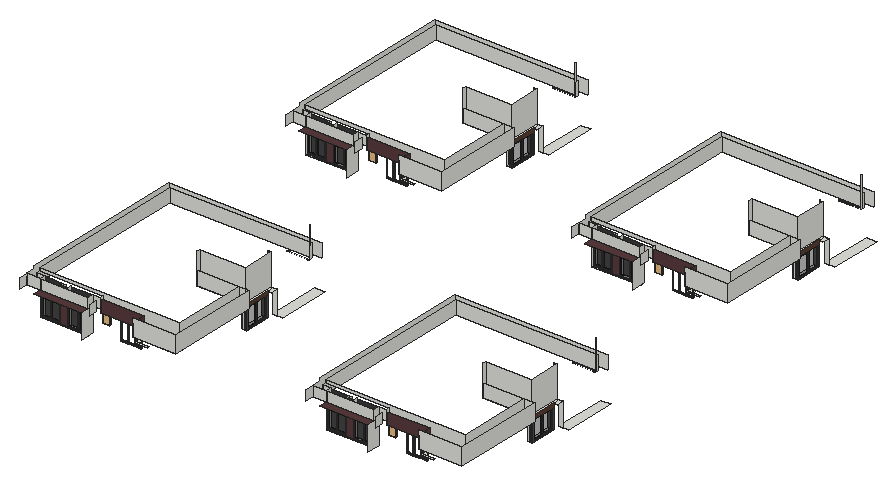
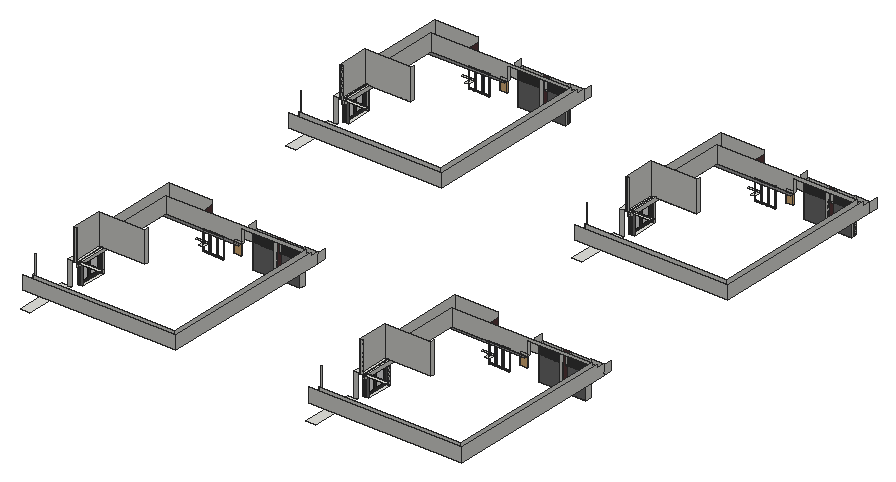
# SketchUp Ruby script. Lengths in inches.
U = 1.inch
M = Sketchup.active_model
def pt(a) = Geom::Point3d.new(a.map { |v| v * U })
def face(e, loops, mat)
  f = e.add_face(loops[0].map { |a| pt(a) })
  loops[1..].each { |l| e.add_face(l.map { |a| pt(a) }).erase! }
  f.material = f.back_material = mat if mat
  f
end
# faces: each face lists its corners as indices into pts; further lists are holes
def faces(e, pts, list, mat = nil) = list.each { |f| face(e, (f[0].is_a?(Array) ? f : [f]).map { |l| l.map { |i| pts[i] } }, mat) }
# xy, xz, yz: faces in a plane at the given z, y or x. An outline is a flat list of corners, or four numbers for a rectangle; further outlines are holes
def ring(l) = l.size == 4 ? [[l[0], l[1]], [l[2], l[1]], [l[2], l[3]], [l[0], l[3]]] : l.each_slice(2).to_a
def flat(e, list, mat, &to3) = list.each { |f| face(e, (f[0].is_a?(Array) ? f : [f]).map { |l| ring(l).map { |u, v| to3.(u, v) } }, mat) }
def xy(e, z, list, mat = nil) = flat(e, list, mat) { |x, y| [x, y, z] }
def xz(e, y, list, mat = nil) = flat(e, list, mat) { |x, z| [x, y, z] }
def yz(e, x, list, mat = nil) = flat(e, list, mat) { |y, z| [x, y, z] }
def lines(e, pts, list) = list.each { |a, b| e.add_line(pt(pts[a]), pt(pts[b])) }
# prism: a flat outline (further loops are holes) pulled along v
def prism(e, loops, v, mat = nil)
  f = face(e, loops, mat); d = Geom::Vector3d.new(v.map { |x| x * U })
  f.pushpull(f.normal.samedirection?(d) ? d.length : -d.length)
end
def box(e, o, s, mat = nil) = prism(e, [[o, [o[0] + s[0], o[1], o[2]], [o[0] + s[0], o[1] + s[1], o[2]], [o[0], o[1] + s[1], o[2]]]], [0, 0, s[2]], mat)
def at(x, y, z, deg = 0) = Geom::Transformation.translation(pt([x, y, z])) * Geom::Transformation.rotation(ORIGIN, Z_AXIS, deg.degrees)
def axes(o, x, y, z) = Geom::Transformation.new([*x, 0, *y, 0, *z, 0, *pt(o).to_a, 1])
def part(name) = M.definitions.add(name)
# library, detail: a bought-in or finely detailed component or shape, given as its bounding box
def library(name, o, s) = part(name).tap { |d| box(d.entities, o, s) }
def detail(e, o, s) = box(e.add_group.entities, o, s)
def put(e, d, t, mat = nil) = e.add_instance(d, t).tap { |i| i.material = mat if mat }
def group(e, t, mat = nil) = e.add_group.tap { |g| g.transformation = t; g.material = mat if mat }.entities
root = M.entities
M.materials.add("Glass_Tinted_Gray").color = [0, 0, 0]
M.materials["Glass_Tinted_Gray"].alpha = 0.125
M.materials.add("Wine2").color = [0, 0, 0]
M.materials["Wine2"].alpha = 0
M.materials.add("[0130_Gainsboro]").color = [39, 45, 50]
M.materials.add("[0135_DarkGray]").color = [81, 81, 81]
M.materials.add("[Color M05]").color = [114, 114, 114]
M.materials.add("[Color M06]").color = [86, 86, 86]
M.materials.add("[Color M07]").color = [58, 58, 58]
M.materials.add("[Granite Brown]").color = [89, 59, 61]
M.materials.add("[Granite Brown]1").color = [89, 63, 50]
M.materials.add("[Mirror 02]").color = [229, 229, 229]
M.materials.add("[Terrazzo Light Blue]").color = [196, 214, 227]
c1 = part("PENTEK_RP Fineline 50S_Sliding_DoorCase_E1")
box(c1.entities,[0,0,0],[1.51,3.66,99.27],"[0135_DarkGray]")
c2 = part("PENTEK_RP Fineline 50S_SlidingDooe_Case_E2")
box(c2.entities,[0,0,0],[96.25,3.66,1.51],"[0135_DarkGray]")
c3 = part("pentek_RP Fineline 50S_SlidingDoor_Case")
put(c3.entities,c1,at(97.76,0,0))
put(c3.entities,c2,at(1.51,0,0))
put(c3.entities,c1,at(0,0,0))
put(c3.entities,c2,at(1.51,0,97.76))
c4 = part("PENTEK_RP Fineline 50S_SlidingDoor_GlazingBead_2")
box(c4.entities,[0,0,0],[0.56,0.59,94.39],"[0135_DarkGray]")
c5 = part("PENTEK_RP Fineline 50S_SlidingDoor_Glass")
box(c5.entities,[0,0,0],[46.58,0.16,94.39],"Glass_Tinted_Gray")
c6 = part("PENTEK_RP Fineline 50S_SlidingDoor_GlazingBead")
box(c6.entities,[0,0,0],[45.47,0.59,0.56],"[0135_DarkGray]")
c7 = part("PENTEK_RP Fineline 50S_SlidingDoor_Leaf_E1")
xy(c7.entities,0,[[0,0,0.93,1.97],[0.93,1.57,1.49,1.97]],"[0135_DarkGray]")
xy(c7.entities,96.25,[[0,0,0.93,0,0.93,1.57,1.49,1.57,1.49,1.97,0,1.97]],"[0135_DarkGray]")
xz(c7.entities,0,[[0,0,0.93,96.25]],"[0135_DarkGray]")
xz(c7.entities,1.57,[[0.93,0,1.49,95.32],[0.93,95.32,1.49,96.25]],"[0135_DarkGray]")
xz(c7.entities,1.97,[[0,0,1.49,96.25]],"[0135_DarkGray]")
yz(c7.entities,0,[[0,0,1.97,96.25]],"[0135_DarkGray]")
yz(c7.entities,0.93,[[0,0,1.57,0.93],[0,0.93,1.57,95.32],[0,95.32,1.57,96.25]],"[0135_DarkGray]")
yz(c7.entities,1.49,[[1.57,0,1.97,95.32],[1.57,95.32,1.97,96.25]],"[0135_DarkGray]")
c8 = part("PENTEK_RP Fineline 50S_SlidingDoor_Leaf_E2")
xy(c8.entities,0,[[0,0,0,1.57,0.56,1.57,0.56,1.97,46.02,1.97,46.02,1.57,46.58,1.57,46.58,0]],"[0135_DarkGray]")
xy(c8.entities,0.93,[[0,0,46.58,1.57]],"[0135_DarkGray]")
xy(c8.entities,1.49,[[0.56,1.57,46.02,1.97]],"[0135_DarkGray]")
xz(c8.entities,0,[[0,0,46.58,0.93]],"[0135_DarkGray]")
xz(c8.entities,1.57,[[0,0,0.56,0.93],[46.02,0,46.58,0.93],[0.56,0.93,46.02,1.49]],"[0135_DarkGray]")
xz(c8.entities,1.97,[[0.56,0,46.02,1.49]],"[0135_DarkGray]")
yz(c8.entities,0,[[0,0,1.57,0.93]],"[0135_DarkGray]")
yz(c8.entities,0.56,[[1.57,0,1.97,0.93],[1.57,0.93,1.97,1.49]],"[0135_DarkGray]")
yz(c8.entities,46.02,[[1.57,0,1.97,0.93],[1.57,0.93,1.97,1.49]],"[0135_DarkGray]")
yz(c8.entities,46.58,[[0,0,1.57,0.93]],"[0135_DarkGray]")
c9 = part("PENTEK_RP Fineline S_SlidingDoor_Leaf1")
put(c9.entities,c4,at(0.93,0,0.93))
put(c9.entities,c4,at(46.96,0,0.93))
put(c9.entities,c5,at(1.49,1.42,0.93))
put(c9.entities,c6,at(1.49,0,0.93))
put(c9.entities,c5,at(1.49,0.59,0.93),"[Terrazzo Light Blue]")
put(c9.entities,c7,at(0,0,0))
put(c9.entities,c7,axes([48.44,0,0],[-1,0,0],[0,1,0],[0,0,1]))
put(c9.entities,c8,axes([0.93,0,96.25],[1,0,0],[0,1,0],[0,0,-1]))
put(c9.entities,c8,at(0.93,0,0))
put(c9.entities,c6,at(1.49,0,94.77))
c10 = part("PENTEK_RP Fineline 50S_SlidingDoor_Leaf2")
put(c10.entities,c5,at(1.49,1.42,0.93))
put(c10.entities,c6,at(1.49,0,94.77))
put(c10.entities,c4,at(46.96,0,0.93))
put(c10.entities,c5,at(1.49,0.59,0.93),"[Mirror 02]")
put(c10.entities,c4,at(0.93,0,0.93))
put(c10.entities,c7,at(0,0,0))
put(c10.entities,c7,axes([48.44,0,0],[-1,0,0],[0,1,0],[0,0,1]))
put(c10.entities,c6,at(1.49,0,0.93))
put(c10.entities,c8,axes([0.93,0,96.25],[1,0,0],[0,1,0],[0,0,-1]))
put(c10.entities,c8,at(0.93,0,0))
c11 = part("PENTEK - Slimmest Steel Sliding Door / Window\#1")
put(c11.entities,c3,at(0,-1.88,-0.09))
put(c11.entities,c9,at(1.51,-2.27,1.42))
put(c11.entities,c10,at(49.32,-0.3,1.42))
c12 = part("Framed glazing panel")
xy(c12.entities,0,[[0,-0.98,43.07,0],[0,0,43.07,1.4]],"[0130_Gainsboro]")
xy(c12.entities,0.3,[[0.3,-1.43,42.77,-0.98]],"[0130_Gainsboro]")
xy(c12.entities,2.95,[[2.95,-1.43,40.12,-0.63],[2.95,-0.63,40.12,0],[2.95,0,40.12,0.64],[2.95,0.64,40.12,1.4]],"[0130_Gainsboro]")
xy(c12.entities,3.54,[[3.54,-0.63,39.53,0],[3.54,0,39.53,0.64]],"[0130_Gainsboro]")
xy(c12.entities,111.8125,[[3.54,-0.63,39.53,0],[3.54,0,39.53,0.64]],"[0130_Gainsboro]")
xy(c12.entities,112.4,[[2.95,-1.43,40.12,-0.63],[2.95,-0.63,40.12,0],[2.95,0,40.12,0.64],[2.95,0.64,40.12,1.4]],"[0130_Gainsboro]")
xy(c12.entities,115.05,[[0.3,-1.43,42.77,-0.98]],"[0130_Gainsboro]")
xy(c12.entities,115.35,[[0,-0.98,43.07,0],[0,0,43.07,1.4]],"[0130_Gainsboro]")
xz(c12.entities,-1.43,[[[0.3,0.3,42.77,115.05],[2.95,2.95,40.12,112.4]]],"[0130_Gainsboro]")
xz(c12.entities,-0.98,[[[0,0,43.07,115.35],[0.3,0.3,42.77,115.05]]],"[0130_Gainsboro]")
xz(c12.entities,-0.63,[[[2.95,2.95,40.12,112.4],[3.54,3.54,39.53,111.8125]]],"[0130_Gainsboro]")
xz(c12.entities,0,[[3.54,3.54,39.53,111.8125]],"Wine2")
xz(c12.entities,0,[[[0,0,43.07,115.35],[2.95,2.95,40.12,112.4]],[[2.95,2.95,40.12,112.4],[3.54,3.54,39.53,111.8125]]],"[0130_Gainsboro]")
xz(c12.entities,0.64,[[[2.95,2.95,40.12,112.4],[3.54,3.54,39.53,111.8125]]],"[0130_Gainsboro]")
xz(c12.entities,1.4,[[[0,0,43.07,115.35],[2.95,2.95,40.12,112.4]]],"[0130_Gainsboro]")
yz(c12.entities,0,[[-0.98,0,0,115.35],[0,0,1.4,115.35]],"[0130_Gainsboro]")
yz(c12.entities,0.3,[[-1.43,0.3,-0.98,115.05]],"[0130_Gainsboro]")
yz(c12.entities,2.95,[[-1.43,2.95,-0.63,112.4],[-0.63,2.95,0,112.4],[0,2.95,0.64,112.4],[0.64,2.95,1.4,112.4]],"[0130_Gainsboro]")
yz(c12.entities,3.54,[[-0.63,3.54,0,111.8125],[0,3.54,0.64,111.8125]],"[0130_Gainsboro]")
yz(c12.entities,39.53,[[-0.63,3.54,0,111.8125],[0,3.54,0.64,111.8125]],"[0130_Gainsboro]")
yz(c12.entities,40.12,[[-1.43,2.95,-0.63,112.4],[-0.63,2.95,0,112.4],[0,2.95,0.64,112.4],[0.64,2.95,1.4,112.4]],"[0130_Gainsboro]")
yz(c12.entities,42.77,[[-1.43,0.3,-0.98,115.05]],"[0130_Gainsboro]")
yz(c12.entities,43.07,[[-0.98,0,0,115.35],[0,0,1.4,115.35]],"[0130_Gainsboro]")
c13 = part("Glazed panel assembly")
put(c13.entities,c12,axes([90.57,1.43,0],[1.05148,0,0],[0,1,0],[0,0,1]))
put(c13.entities,c12,axes([0,1.43,0],[1.05148,0,0],[0,1,0],[0,0,1]))
put(c13.entities,c12,axes([45.29,1.43,0],[1.05148,0,0],[0,1,0],[0,0,1]))
c14 = library("Klein+raam",[128.36,12.7,0],[19.68,5.51,55.12])
xy(root,1659.3125,[[319.53,1799.9375,523.04,1799.9375,523.04,1822.9375,431.33,1822.9375,431.33,1806.5625,406.84,1806.5625,406.84,1822.9375,319.53,1822.9375],[1537.72,1799.9375,1741.23,1799.9375,1741.23,1822.9375,1649.52,1822.9375,1649.52,1806.5625,1625.03,1806.5625,1625.03,1822.9375,1537.72,1822.9375],[319.53,3214.625,523.04,3214.625,523.04,3237.625,431.33,3237.625,431.33,3221.25,406.84,3221.25,406.84,3237.625,319.53,3237.625],[1537.72,3214.625,1741.23,3214.625,1741.23,3237.625,1649.52,3237.625,1649.52,3221.25,1625.03,3221.25,1625.03,3237.625,1537.72,3237.625]])
xy(root,1661.36,[[890.875,2156.01,913.875,2266.33],[2109.0625,2156.01,2132.0625,2266.33],[890.875,3570.7,913.875,3681.01],[2109.0625,3570.7,2132.0625,3681.01]])
xy(root,1663.0625,[[913.875,2295.875,954.6875,2518.89],[2132.0625,2295.875,2172.875,2518.89],[913.875,3710.5625,954.6875,3933.57],[2132.0625,3710.5625,2172.875,3933.57]])
xy(root,1693.1875,[[709.36,1814.25,764.59,1822.9375],[1927.54,1814.25,1982.78,1822.9375],[709.01,1822.9375,727.9,1851.6875],[1927.2,1822.9375,1946.09,1851.6875],[709.36,3228.9375,764.59,3237.625],
  [1927.54,3228.9375,1982.78,3237.625],[709.01,3237.625,727.9,3266.375],[1927.2,3237.625,1946.09,3266.375]])
xy(root,1747,[[894.3125,2107.9375,913.875,2148.625],[2112.5,2107.9375,2132.0625,2148.625],[894.3125,3522.625,913.875,3563.3125],[2112.5,3522.625,2132.0625,3563.3125]])
xy(root,1747.04,[[894.3125,2148.83,913.875,2156.01],[2112.5,2148.83,2132.0625,2156.01],[890.875,2156.01,913.875,2266.33],[2109.0625,2156.01,2132.0625,2266.33],[894.3125,3563.51,913.875,3570.7],
  [2112.5,3563.51,2132.0625,3570.7],[890.875,3570.7,913.875,3681.01],[2109.0625,3570.7,2132.0625,3681.01]])
xy(root,1749.375,[[883.05,1851.6875,894.3125,2295.875],[2101.24,1851.6875,2112.5,2295.875],[883.05,3266.375,894.3125,3710.5625],[2101.24,3266.375,2112.5,3710.5625]])
xy(root,1749.375,[[557.88,1835.8125,883.05,1851.6875],[1776.07,1835.8125,2101.24,1851.6875],[557.88,3250.5,883.05,3266.375],[1776.07,3250.5,2101.24,3266.375]],"[Color M05]")
xy(root,1749.375,[[741.54,1763.25,925.6875,1799.9375],[1959.73,1763.25,2143.875,1799.9375],[741.54,1799.9375,925.6875,1822.9375],[1959.73,1799.9375,2143.875,1822.9375],[557.88,1822.9375,557.88,1835.8125,883.05,1835.8125,883.05,1851.6875,894.3125,1851.6875,894.3125,2148.83,925.6875,2148.83,925.6875,1822.9375],
  [1776.07,1822.9375,1776.07,1835.8125,2101.24,1835.8125,2101.24,1851.6875,2112.5,1851.6875,2112.5,2148.83,2143.875,2148.83,2143.875,1822.9375],[557.4,1835.1875,557.88,1835.8125],[1775.59,1835.1875,1776.07,1835.8125],[741.54,3177.9375,925.6875,3214.625],[1959.73,3177.9375,2143.875,3214.625],
  [741.54,3214.625,925.6875,3237.625],[1959.73,3214.625,2143.875,3237.625],[557.88,3237.625,557.88,3250.5,883.05,3250.5,883.05,3266.375,894.3125,3266.375,894.3125,3563.51,925.6875,3563.51,925.6875,3237.625],[1776.07,3237.625,1776.07,3250.5,2101.24,3250.5,2101.24,3266.375,2112.5,3266.375,2112.5,3563.51,2143.875,3563.51,2143.875,3237.625],[557.4,3249.875,557.88,3250.5],
  [1775.59,3249.875,1776.07,3250.5]],"[Color M06]")
xy(root,1749.375,[[557.4,1822.9375,557.88,1835.1875],[1775.59,1822.9375,1776.07,1835.1875],[557.4,3237.625,557.88,3249.875],[1775.59,3237.625,1776.07,3249.875]],"[Granite Brown]")
xy(root,1764,[[890.875,1835.8125,894.3125,2148.83],[2109.0625,1835.8125,2112.5,2148.83],[708.18,2148.83,883.05,2162.73],[883.05,2148.83,890.875,2162.73],[890.875,2148.83,894.3125,2162.73],
  [894.3125,2148.83,913.875,2148.83,913.875,2295.875,903.5,2295.875,903.5,2162.73,894.3125,2162.73],[1926.36,2148.83,2101.24,2162.73],[2101.24,2148.83,2109.0625,2162.73],[2109.0625,2148.83,2112.5,2162.73],[2112.5,2148.83,2132.0625,2148.83,2132.0625,2295.875,2121.6875,2295.875,2121.6875,2162.73,2112.5,2162.73],
  [883.05,2162.73,890.875,2278.25],[890.875,2162.73,894.3125,2295.875],[894.3125,2162.73,903.5,2295.875],[2101.24,2162.73,2109.0625,2278.25],[2109.0625,2162.73,2112.5,2295.875],
  [2112.5,2162.73,2121.6875,2295.875],[913.875,2266.33,930.75,2295.875],[2132.0625,2266.33,2148.9375,2295.875],[795.3125,2278.25,883.05,2284.4375],[883.05,2278.25,890.875,2284.4375],
  [2013.5,2278.25,2101.24,2284.4375],[2101.24,2278.25,2109.0625,2284.4375],[795.3125,2284.4375,883.05,2295.875],[883.05,2284.4375,890.875,2295.875],[2013.5,2284.4375,2101.24,2295.875],
  [2101.24,2284.4375,2109.0625,2295.875],[795.3125,2517.14,890.875,2518.89],[2013.5,2517.14,2109.0625,2518.89],[890.875,3250.5,894.3125,3563.51],[2109.0625,3250.5,2112.5,3563.51],
  [708.18,3563.51,883.05,3577.41],[883.05,3563.51,890.875,3577.41],[890.875,3563.51,894.3125,3577.41],[894.3125,3563.51,913.875,3563.51,913.875,3710.5625,903.5,3710.5625,903.5,3577.41,894.3125,3577.41],[1926.36,3563.51,2101.24,3577.41],
  [2101.24,3563.51,2109.0625,3577.41],[2109.0625,3563.51,2112.5,3577.41],[2112.5,3563.51,2132.0625,3563.51,2132.0625,3710.5625,2121.6875,3710.5625,2121.6875,3577.41,2112.5,3577.41],[883.05,3577.41,890.875,3692.9375],[890.875,3577.41,894.3125,3710.5625],
  [894.3125,3577.41,903.5,3710.5625],[2101.24,3577.41,2109.0625,3692.9375],[2109.0625,3577.41,2112.5,3710.5625],[2112.5,3577.41,2121.6875,3710.5625],[913.875,3681.01,930.75,3710.5625],
  [2132.0625,3681.01,2148.9375,3710.5625],[795.3125,3692.9375,883.05,3699.125],[883.05,3692.9375,890.875,3699.125],[2013.5,3692.9375,2101.24,3699.125],[2101.24,3692.9375,2109.0625,3699.125],
  [795.3125,3699.125,883.05,3710.5625],[883.05,3699.125,890.875,3710.5625],[2013.5,3699.125,2101.24,3710.5625],[2101.24,3699.125,2109.0625,3710.5625],[795.3125,3931.82,890.875,3933.57],
  [2013.5,3931.82,2109.0625,3933.57]])
xy(root,1764,[[319.53,1763.25,523.04,1799.9375],[1537.72,1763.25,1741.23,1799.9375],[319.53,3177.9375,523.04,3214.625],[1537.72,3177.9375,1741.23,3214.625]],"[Granite Brown]")
xz(root,1763.25,[[741.54,1749.375,925.6875,1821.625],[1959.73,1749.375,2143.875,1821.625]])
xz(root,1763.25,[[557.4,1764,557.88,1801.625],[1775.59,1764,1776.07,1801.625]],"[Granite Brown]")
xz(root,1799.9375,[[262.875,1764,319.53,1807.33],[319.53,1764,523.04,1805.3125],[1481.0625,1764,1537.72,1807.33],[1537.72,1764,1741.23,1805.3125]])
xz(root,1806.5625,[[406.84,1659.3125,431.33,1659.3125,431.33,1808.75,407.44,1808.75,407.44,1805.3125,396.84,1805.37,396.63,1764.05,396.11,1659.37],[1625.03,1659.3125,1649.52,1659.3125,1649.52,1808.75,1625.63,1808.75,1625.63,1805.3125,1615.02,1805.37,1614.82,1764.05,1614.29,1659.37]],"[Granite Brown]")
xz(root,1822.9375,[[285.875,1764,319.53,1807.33],[396.63,1764,396.84,1764.05],[396.84,1764,396.84,1764.05,407.44,1764],[407.44,1764,396.84,1764.05,396.84,1805.37,407.44,1805.3125],[407.44,1764,407.44,1805.3125,407.65,1805.3125],
  [523.04,1764,557.4,1805.3125],[1504.0625,1764,1537.72,1807.33],[1614.82,1764,1615.02,1764.05],[1615.02,1764,1615.02,1764.05,1625.63,1764],[1625.63,1764,1615.02,1764.05,1615.02,1805.37,1625.63,1805.3125],
  [1625.63,1764,1625.63,1805.3125,1625.84,1805.3125],[1741.23,1764,1775.59,1805.3125],[396.63,1764.05,396.84,1805.37,396.84,1764.05],[1614.82,1764.05,1615.02,1805.37,1615.02,1764.05]])
xz(root,1822.9375,[[319.53,1659.3125,396.11,1659.3125,396.63,1764,319.53,1764],[431.33,1659.3125,523.04,1764],[1537.72,1659.3125,1614.29,1659.3125,1614.82,1764,1537.72,1764],[1649.52,1659.3125,1741.23,1764]],"[Color M05]")
xz(root,1822.9375,[[319.53,1764,319.53,1805.37,396.84,1805.37,396.63,1764.05,396.63,1764],[431.33,1764,523.04,1805.3125],[1537.72,1764,1537.72,1805.37,1615.02,1805.37,1614.82,1764.05,1614.82,1764],[1649.52,1764,1741.23,1805.3125]],"[Color M07]")
xz(root,1822.9375,[[557.4,1749.375,557.88,1764],[557.88,1749.375,741.54,1801.625],[1775.59,1749.375,1776.07,1764],[1776.07,1749.375,1959.73,1801.625],[557.4,1764,557.88,1801.625],
  [1775.59,1764,1776.07,1801.625]],"[Granite Brown]")
xz(root,1835.1875,[[556.34,1706.43,557.4,1758.71],[1774.53,1706.43,1775.59,1758.71]])
xz(root,1835.8125,[[557.4,1749.375,557.4,1807.33,285.875,1807.33,285.875,1821.625,883.05,1821.625,883.05,1749.375],[1775.59,1749.375,1775.59,1807.33,1504.0625,1807.33,1504.0625,1821.625,2101.24,1821.625,2101.24,1749.375]])
xz(root,2148.83,[[894.3125,1747.04,913.875,1749.375],[2112.5,1747.04,2132.0625,1749.375],[913.875,1749.375,925.6875,1764],[2132.0625,1749.375,2143.875,1764],[708.18,1764,883.05,1821.625],
  [883.05,1764,913.875,1821.625],[913.875,1764,925.6875,1821.625],[1926.36,1764,2101.24,1821.625],[2101.24,1764,2132.0625,1821.625],[2132.0625,1764,2143.875,1821.625]])
xz(root,2156.01,[[890.875,1661.36,894.3125,1747.04],[894.3125,1661.36,913.875,1747.04],[2109.0625,1661.36,2112.5,1747.04],[2112.5,1661.36,2132.0625,1747.04]])
xz(root,2162.73,[[708.18,1764,903.5,1895.25],[1926.36,1764,2121.6875,1895.25]])
xz(root,2266.33,[[890.875,1661.36,913.875,1747.04],[2109.0625,1661.36,2132.0625,1747.04]],"[Color M05]")
xz(root,2295.875,[[913.875,1663.0625,930.75,1764],[2132.0625,1663.0625,2148.9375,1764],[883.05,1749.375,890.875,1764],[890.875,1749.375,894.3125,1764],[2101.24,1749.375,2109.0625,1764],
  [2109.0625,1749.375,2112.5,1764],[890.875,1764,894.3125,1895.25],[894.3125,1764,903.5,1895.25],[2109.0625,1764,2112.5,1895.25],[2112.5,1764,2121.6875,1895.25]])
xz(root,2531.375,[[285.875,1764,890.875,1821.625],[1504.0625,1764,2109.0625,1821.625]])
xz(root,2554.375,[[262.875,1764,913.875,1821.625],[1481.0625,1764,2132.0625,1821.625]])
xz(root,3177.9375,[[741.54,1749.375,925.6875,1821.625],[1959.73,1749.375,2143.875,1821.625]])
xz(root,3177.9375,[[557.4,1764,557.88,1801.625],[1775.59,1764,1776.07,1801.625]],"[Granite Brown]")
xz(root,3214.625,[[262.875,1764,319.53,1807.33],[319.53,1764,523.04,1805.3125],[1481.0625,1764,1537.72,1807.33],[1537.72,1764,1741.23,1805.3125]])
xz(root,3221.25,[[406.84,1659.3125,431.33,1659.3125,431.33,1808.75,407.44,1808.75,407.44,1805.3125,396.84,1805.37,396.63,1764.05,396.11,1659.37],[1625.03,1659.3125,1649.52,1659.3125,1649.52,1808.75,1625.63,1808.75,1625.63,1805.3125,1615.02,1805.37,1614.82,1764.05,1614.29,1659.37]],"[Granite Brown]")
xz(root,3237.625,[[285.875,1764,319.53,1807.33],[396.63,1764,396.84,1764.05],[396.84,1764,396.84,1764.05,407.44,1764],[407.44,1764,396.84,1764.05,396.84,1805.37,407.44,1805.3125],[407.44,1764,407.44,1805.3125,407.65,1805.3125],
  [523.04,1764,557.4,1805.3125],[1504.0625,1764,1537.72,1807.33],[1614.82,1764,1615.02,1764.05],[1615.02,1764,1615.02,1764.05,1625.63,1764],[1625.63,1764,1615.02,1764.05,1615.02,1805.37,1625.63,1805.3125],
  [1625.63,1764,1625.63,1805.3125,1625.84,1805.3125],[1741.23,1764,1775.59,1805.3125],[396.63,1764.05,396.84,1805.37,396.84,1764.05],[1614.82,1764.05,1615.02,1805.37,1615.02,1764.05]])
xz(root,3237.625,[[319.53,1659.3125,396.11,1659.3125,396.63,1764,319.53,1764],[431.33,1659.3125,523.04,1764],[1537.72,1659.3125,1614.29,1659.3125,1614.82,1764,1537.72,1764],[1649.52,1659.3125,1741.23,1764]],"[Color M05]")
xz(root,3237.625,[[319.53,1764,319.53,1805.37,396.84,1805.37,396.63,1764.05,396.63,1764],[431.33,1764,523.04,1805.3125],[1537.72,1764,1537.72,1805.37,1615.02,1805.37,1614.82,1764.05,1614.82,1764],[1649.52,1764,1741.23,1805.3125]],"[Color M07]")
xz(root,3237.625,[[557.4,1749.375,557.88,1764],[557.88,1749.375,741.54,1801.625],[1775.59,1749.375,1776.07,1764],[1776.07,1749.375,1959.73,1801.625],[557.4,1764,557.88,1801.625],
  [1775.59,1764,1776.07,1801.625]],"[Granite Brown]")
xz(root,3249.875,[[556.34,1706.43,557.4,1758.71],[1774.53,1706.43,1775.59,1758.71]])
xz(root,3250.5,[[557.4,1749.375,557.4,1807.33,285.875,1807.33,285.875,1821.625,883.05,1821.625,883.05,1749.375],[1775.59,1749.375,1775.59,1807.33,1504.0625,1807.33,1504.0625,1821.625,2101.24,1821.625,2101.24,1749.375]])
xz(root,3563.51,[[894.3125,1747.04,913.875,1749.375],[2112.5,1747.04,2132.0625,1749.375],[913.875,1749.375,925.6875,1764],[2132.0625,1749.375,2143.875,1764],[708.18,1764,883.05,1821.625],
  [883.05,1764,913.875,1821.625],[913.875,1764,925.6875,1821.625],[1926.36,1764,2101.24,1821.625],[2101.24,1764,2132.0625,1821.625],[2132.0625,1764,2143.875,1821.625]])
xz(root,3570.7,[[890.875,1661.36,894.3125,1747.04],[894.3125,1661.36,913.875,1747.04],[2109.0625,1661.36,2112.5,1747.04],[2112.5,1661.36,2132.0625,1747.04]])
xz(root,3577.41,[[708.18,1764,903.5,1895.25],[1926.36,1764,2121.6875,1895.25]])
xz(root,3681.01,[[890.875,1661.36,913.875,1747.04],[2109.0625,1661.36,2132.0625,1747.04]],"[Color M05]")
xz(root,3710.5625,[[913.875,1663.0625,930.75,1764],[2132.0625,1663.0625,2148.9375,1764],[883.05,1749.375,890.875,1764],[890.875,1749.375,894.3125,1764],[2101.24,1749.375,2109.0625,1764],
  [2109.0625,1749.375,2112.5,1764],[890.875,1764,894.3125,1895.25],[894.3125,1764,903.5,1895.25],[2109.0625,1764,2112.5,1895.25],[2112.5,1764,2121.6875,1895.25]])
xz(root,3946.0625,[[285.875,1764,890.875,1821.625],[1504.0625,1764,2109.0625,1821.625]])
xz(root,3969.0625,[[262.875,1764,913.875,1821.625],[1481.0625,1764,2132.0625,1821.625]])
yz(root,262.875,[[1763.25,1764,1799.9375,1805.3125],[1799.9375,1764,1799.9375,1807.33,1835.8125,1807.33,1835.8125,1821.625,2554.375,1821.625,2554.375,1764],[3177.9375,1764,3214.625,1805.3125],[3214.625,1764,3214.625,1807.33,3250.5,1807.33,3250.5,1821.625,3969.0625,1821.625,3969.0625,1764]])
yz(root,285.875,[[1822.9375,1764,2531.375,1764,2531.375,1821.625,1835.8125,1821.625,1835.8125,1807.33,1822.9375,1807.33],[3237.625,1764,3946.0625,1764,3946.0625,1821.625,3250.5,1821.625,3250.5,1807.33,3237.625,1807.33]])
yz(root,319.53,[[1799.9375,1659.3125,1822.9375,1764],[3214.625,1659.3125,3237.625,1764],[1799.9375,1764,1822.9375,1807.33],[3214.625,1764,3237.625,1807.33]])
yz(root,431.33,[[1806.5625,1659.3125,1822.9375,1808.75],[3221.25,1659.3125,3237.625,1808.75]])
yz(root,523.04,[[1763.25,1659.3125,1822.9375,1764],[3177.9375,1659.3125,3237.625,1764],[1799.9375,1764,1822.9375,1805.3125],[3214.625,1764,3237.625,1805.3125]])
yz(root,557.22,[[1763.25,1764,1799.9375,1805.3125],[3177.9375,1764,3214.625,1805.3125]])
yz(root,557.4,[[1822.9375,1749.375,1835.8125,1807.33],[3237.625,1749.375,3250.5,1807.33]])
yz(root,708.18,[[2148.83,1764,2162.73,1895.25],[3563.51,1764,3577.41,1895.25]])
yz(root,741.54,[[1763.25,1749.375,1799.9375,1801.625],[1799.9375,1749.375,1822.9375,1801.625],[3177.9375,1749.375,3214.625,1801.625],[3214.625,1749.375,3237.625,1801.625]],"[Granite Brown]")
yz(root,883.05,[[1835.8125,1749.375,1835.8125,1821.625,2148.83,1821.625,2148.83,1764,2295.875,1764,2295.875,1749.375],[3250.5,1749.375,3250.5,1821.625,3563.51,1821.625,3563.51,1764,3710.5625,1764,3710.5625,1749.375]])
yz(root,890.875,[[2517.14,1764,2518.89,1895.25],[2518.89,1764,2531.375,1821.625],[3931.82,1764,3933.57,1895.25],[3933.57,1764,3946.0625,1821.625]])
yz(root,894.3125,[[2148.83,1749.375,2295.875,1764],[3563.51,1749.375,3710.5625,1764]])
yz(root,903.5,[[2162.73,1764,2295.875,1895.25],[3577.41,1764,3710.5625,1895.25]])
yz(root,913.875,[[2148.83,1747.04,2266.33,1764],[3563.51,1747.04,3681.01,1764]],"[Granite Brown]1")
yz(root,925.6875,[[1763.25,1749.375,2148.83,1821.625],[3177.9375,1749.375,3563.51,1821.625]])
yz(root,1481.0625,[[1763.25,1764,1799.9375,1805.3125],[1799.9375,1764,1799.9375,1807.33,1835.8125,1807.33,1835.8125,1821.625,2554.375,1821.625,2554.375,1764],[3177.9375,1764,3214.625,1805.3125],[3214.625,1764,3214.625,1807.33,3250.5,1807.33,3250.5,1821.625,3969.0625,1821.625,3969.0625,1764]])
yz(root,1504.0625,[[1822.9375,1764,2531.375,1764,2531.375,1821.625,1835.8125,1821.625,1835.8125,1807.33,1822.9375,1807.33],[3237.625,1764,3946.0625,1764,3946.0625,1821.625,3250.5,1821.625,3250.5,1807.33,3237.625,1807.33]])
yz(root,1537.72,[[1799.9375,1659.3125,1822.9375,1764],[3214.625,1659.3125,3237.625,1764],[1799.9375,1764,1822.9375,1807.33],[3214.625,1764,3237.625,1807.33]])
yz(root,1649.52,[[1806.5625,1659.3125,1822.9375,1808.75],[3221.25,1659.3125,3237.625,1808.75]])
yz(root,1741.23,[[1763.25,1659.3125,1822.9375,1764],[3177.9375,1659.3125,3237.625,1764],[1799.9375,1764,1822.9375,1805.3125],[3214.625,1764,3237.625,1805.3125]])
yz(root,1775.4,[[1763.25,1764,1799.9375,1805.3125],[3177.9375,1764,3214.625,1805.3125]])
yz(root,1775.59,[[1822.9375,1749.375,1835.8125,1807.33],[3237.625,1749.375,3250.5,1807.33]])
yz(root,1926.36,[[2148.83,1764,2162.73,1895.25],[3563.51,1764,3577.41,1895.25]])
yz(root,1959.73,[[1763.25,1749.375,1799.9375,1801.625],[1799.9375,1749.375,1822.9375,1801.625],[3177.9375,1749.375,3214.625,1801.625],[3214.625,1749.375,3237.625,1801.625]],"[Granite Brown]")
yz(root,2101.24,[[1835.8125,1749.375,1835.8125,1821.625,2148.83,1821.625,2148.83,1764,2295.875,1764,2295.875,1749.375],[3250.5,1749.375,3250.5,1821.625,3563.51,1821.625,3563.51,1764,3710.5625,1764,3710.5625,1749.375]])
yz(root,2109.0625,[[2517.14,1764,2518.89,1895.25],[2518.89,1764,2531.375,1821.625],[3931.82,1764,3933.57,1895.25],[3933.57,1764,3946.0625,1821.625]])
yz(root,2112.5,[[2148.83,1749.375,2295.875,1764],[3563.51,1749.375,3710.5625,1764]])
yz(root,2121.6875,[[2162.73,1764,2295.875,1895.25],[3577.41,1764,3710.5625,1895.25]])
yz(root,2132.0625,[[2148.83,1747.04,2266.33,1764],[3563.51,1747.04,3681.01,1764]],"[Granite Brown]1")
yz(root,2143.875,[[1763.25,1749.375,2148.83,1821.625],[3177.9375,1749.375,3563.51,1821.625]])
p = [[396.63,1822.9375,1764.05],[396.63,1806.5625,1764.05],[396.84,1806.5625,1805.37],[396.84,1822.9375,1805.37],[1614.82,1822.9375,1764.05],[1614.82,1806.5625,1764.05],
  [1615.02,1806.5625,1805.37],[1615.02,1822.9375,1805.37],[396.63,3237.625,1764.05],[396.63,3221.25,1764.05],[396.84,3221.25,1805.37],[396.84,3237.625,1805.37],
  [1614.82,3237.625,1764.05],[1614.82,3221.25,1764.05],[1615.02,3221.25,1805.37],[1615.02,3237.625,1805.37],[1806.84,1835.1875,1706.43],[1806.84,1835.1875,1758.71],
  [1775.59,1835.1875,1706.43],[1775.59,1835.1875,1758.71],[1625.63,1806.5625,1764],[1625.63,1822.9375,1764],[588.66,1835.1875,1706.43],[588.66,1835.1875,1758.71],
  [557.4,1835.1875,1706.43],[557.4,1835.1875,1758.71],[407.44,1806.5625,1764],[407.44,1822.9375,1764],[1625.63,3221.25,1764],[1625.63,3237.625,1764],
  [1775.59,3249.875,1706.43],[1806.84,3249.875,1706.43],[1806.84,3249.875,1758.71],[1775.59,3249.875,1758.71],[557.4,3249.875,1706.43],[588.66,3249.875,1706.43],
  [588.66,3249.875,1758.71],[557.4,3249.875,1758.71],[407.44,3221.25,1764],[407.44,3237.625,1764]]
faces(root,p,[[0,1,2,3],[4,5,6,7],[8,9,10,11],[12,13,14,15]])
lines(root,p,[[16,17],[18,16],[17,19],[20,21],[22,23],[24,22],[23,25],[26,27],[28,29],[30,31],[31,32],[32,33],
  [34,35],[35,36],[36,37],[38,39]])
put(root,c11,axes([1649.52,1806.5625,1659.3125],[0.92378,0,0],[0,1,0],[0,0,1.054]))
put(root,c11,axes([431.33,1806.5625,1659.3125],[0.92378,0,0],[0,1,0],[0,0,1.054]))
put(root,c11,axes([1649.52,3221.25,1659.3125],[0.92378,0,0],[0,1,0],[0,0,1.054]))
put(root,c11,axes([431.33,3221.25,1659.3125],[0.92378,0,0],[0,1,0],[0,0,1.054]))
put(root,c11,axes([1537.72,1808.83,1659.46],[0.7714,0,0],[0,1,0],[0,0,1.054]))
put(root,c11,axes([319.53,1808.83,1659.46],[0.7714,0,0],[0,1,0],[0,0,1.054]))
put(root,c11,axes([1537.72,3223.52,1659.46],[0.7714,0,0],[0,1,0],[0,0,1.054]))
put(root,c11,axes([319.53,3223.52,1659.46],[0.7714,0,0],[0,1,0],[0,0,1.054]))
put(root,c11,axes([2126.35,2154.96,1661.4375],[0,1.12181,0],[-2.51374,0,0],[0,0,0.87918]))
put(root,c11,axes([908.17,2154.96,1661.4375],[0,1.12181,0],[-2.51374,0,0],[0,0,0.87918]))
put(root,c11,axes([2126.35,3569.65,1661.4375],[0,1.12181,0],[-2.51374,0,0],[0,0,0.87918]))
put(root,c11,axes([908.17,3569.65,1661.4375],[0,1.12181,0],[-2.51374,0,0],[0,0,0.87918]))
put(root,c13,axes([1851.32,1835.1875,1664.72],[0.6649,0,0],[0,0.61,0],[0,0,0.74986]),"[Color M06]")
put(root,c13,axes([633.13,1835.1875,1664.72],[0.6649,0,0],[0,0.61,0],[0,0,0.74986]),"[Color M06]")
put(root,c13,axes([1851.32,3249.875,1664.72],[0.6649,0,0],[0,0.61,0],[0,0,0.74986]),"[Color M06]")
put(root,c13,axes([633.13,3249.875,1664.72],[0.6649,0,0],[0,0.61,0],[0,0,0.74986]),"[Color M06]")
put(root,c14,axes([1571.78,1826.29,1706.43],[1.58777,0,0],[0,0.68,0],[0,0,0.7684]))
put(root,c14,axes([353.6,1826.29,1706.43],[1.58777,0,0],[0,0.68,0],[0,0,0.7684]))
put(root,c14,axes([1571.78,3240.97,1706.43],[1.58777,0,0],[0,0.68,0],[0,0,0.7684]))
put(root,c14,axes([353.6,3240.97,1706.43],[1.58777,0,0],[0,0.68,0],[0,0,0.7684]))
